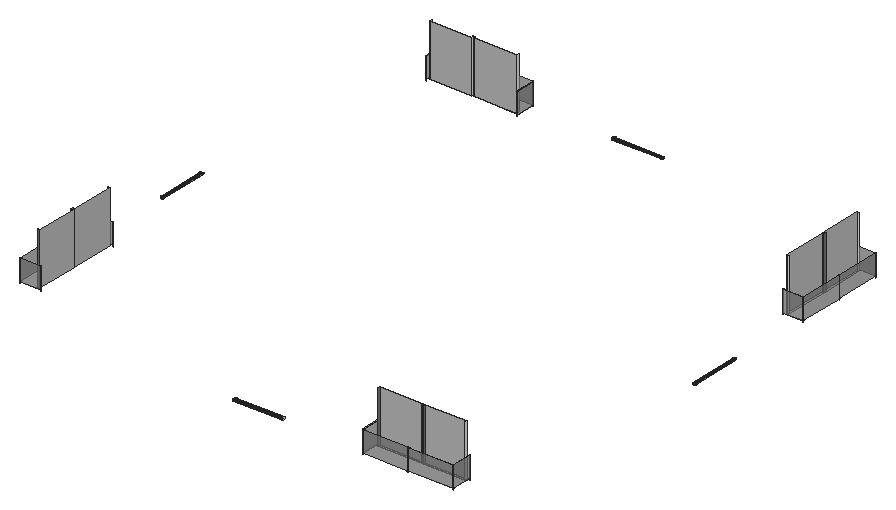
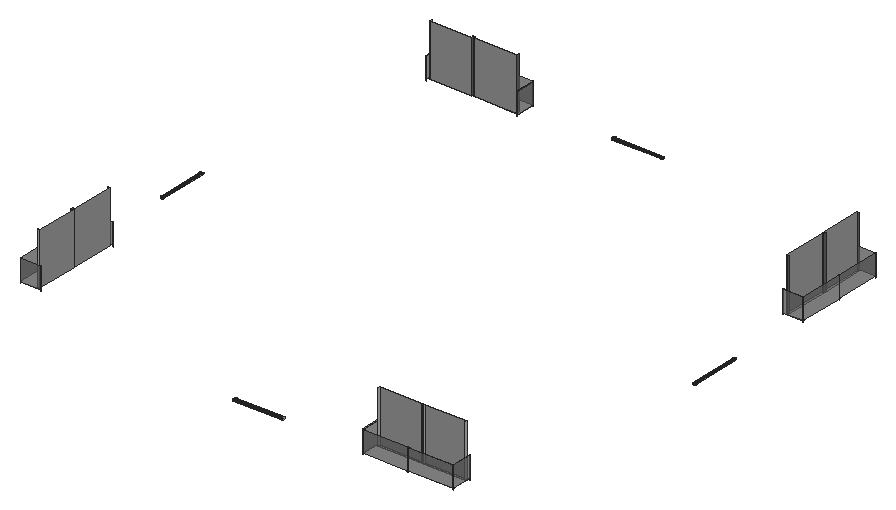
# SketchUp Ruby script. Lengths in inches.
U = 1.inch
M = Sketchup.active_model
def pt(a) = Geom::Point3d.new(a.map { |v| v * U })
def face(e, loops, mat)
  f = e.add_face(loops[0].map { |a| pt(a) })
  loops[1..].each { |l| e.add_face(l.map { |a| pt(a) }).erase! }
  f.material = f.back_material = mat if mat
  f
end
# faces: each face lists its corners as indices into pts; further lists are holes
def faces(e, pts, list, mat = nil) = list.each { |f| face(e, (f[0].is_a?(Array) ? f : [f]).map { |l| l.map { |i| pts[i] } }, mat) }
# xy, xz, yz: faces in a plane at the given z, y or x. An outline is a flat list of corners, or four numbers for a rectangle; further outlines are holes
def ring(l) = l.size == 4 ? [[l[0], l[1]], [l[2], l[1]], [l[2], l[3]], [l[0], l[3]]] : l.each_slice(2).to_a
def flat(e, list, mat, &to3) = list.each { |f| face(e, (f[0].is_a?(Array) ? f : [f]).map { |l| ring(l).map { |u, v| to3.(u, v) } }, mat) }
def xy(e, z, list, mat = nil) = flat(e, list, mat) { |x, y| [x, y, z] }
def xz(e, y, list, mat = nil) = flat(e, list, mat) { |x, z| [x, y, z] }
def yz(e, x, list, mat = nil) = flat(e, list, mat) { |y, z| [x, y, z] }
def lines(e, pts, list) = list.each { |a, b| e.add_line(pt(pts[a]), pt(pts[b])) }
# prism: a flat outline (further loops are holes) pulled along v
def prism(e, loops, v, mat = nil)
  f = face(e, loops, mat); d = Geom::Vector3d.new(v.map { |x| x * U })
  f.pushpull(f.normal.samedirection?(d) ? d.length : -d.length)
end
def box(e, o, s, mat = nil) = prism(e, [[o, [o[0] + s[0], o[1], o[2]], [o[0] + s[0], o[1] + s[1], o[2]], [o[0], o[1] + s[1], o[2]]]], [0, 0, s[2]], mat)
def at(x, y, z, deg = 0) = Geom::Transformation.translation(pt([x, y, z])) * Geom::Transformation.rotation(ORIGIN, Z_AXIS, deg.degrees)
def axes(o, x, y, z) = Geom::Transformation.new([*x, 0, *y, 0, *z, 0, *pt(o).to_a, 1])
def part(name) = M.definitions.add(name)
# library, detail: a bought-in or finely detailed component or shape, given as its bounding box
def library(name, o, s) = part(name).tap { |d| box(d.entities, o, s) }
def detail(e, o, s) = box(e.add_group.entities, o, s)
def put(e, d, t, mat = nil) = e.add_instance(d, t).tap { |i| i.material = mat if mat }
def group(e, t, mat = nil) = e.add_group.tap { |g| g.transformation = t; g.material = mat if mat }.entities
root = M.entities
M.materials.add("[Metal Seamed]").color = [118, 119, 115]
M.materials.add("[Mirror 01]").color = [185, 185, 185]
M.materials.add("[Translucent Glass Tinted]").color = [8, 201, 241]
M.materials["[Translucent Glass Tinted]"].alpha = 0.48
M.materials.add("[Translucent_Glass_Gray]").color = [128, 128, 128]
M.materials["[Translucent_Glass_Gray]"].alpha = 0.5
c1 = part("Staal sojle alta")
box(c1.entities,[0,0,0],[0.87,0.87,43.31])
c2 = part("gler")
box(c2.entities,[0,-0.71,0],[0.37,57.8,41.34],"[Translucent_Glass_Gray]")
xy(root,859.11,[[1161.2,84.8125,1285.04,90.8125],[1291.04,84.8125,1408.89,90.8125],[120,175.92,126,293.77],[120,299.77,126,423.61],[1494,1126.01,1500,1249.86],
  [1494,1255.86,1500,1373.7],[211.11,1458.8125,328.96,1464.8125],[334.96,1458.8125,458.8,1464.8125]])
xz(root,84.8125,[[1285.04,859.11,1291.04,1007.61]],"[Metal Seamed]")
xz(root,90.8125,[[1161.2,859.11,1285.04,1007.61],[1291.04,859.11,1408.89,1007.61]],"[Mirror 01]")
xz(root,175.92,[[120,859.11,126,1007.61]],"[Metal Seamed]")
xz(root,293.77,[[120,859.11,126,1007.61]],"[Metal Seamed]")
xz(root,299.77,[[120,859.11,126,1007.61]],"[Metal Seamed]")
xz(root,423.61,[[120,859.11,126,1007.61]],"[Metal Seamed]")
xz(root,662.8,[[83.53,858.02,84.48,858.14,85.37,858.51,86.13,859.1,86.72,859.86,87.09,860.75,87.21,861.7,87.09,862.66,86.72,863.55,86.13,864.3125,85.37,864.9,84.48,865.27,83.53,865.39,82.57,865.27,81.68,864.9,80.92,864.3125,80.33,863.55,79.97,862.66,79.84,861.7,79.97,860.75,80.33,859.86,80.92,859.1,81.68,858.51,82.57,858.14]])
xz(root,886.83,[[1536.47,858.02,1535.52,858.14,1534.63,858.51,1533.87,859.1,1533.28,859.86,1532.91,860.75,1532.79,861.7,1532.91,862.66,1533.28,863.55,1533.87,864.3125,1534.63,864.9,1535.52,865.27,1536.47,865.39,1537.43,865.27,1538.32,864.9,1539.08,864.3125,1539.67,863.55,1540.03,862.66,1540.16,861.7,1540.03,860.75,1539.67,859.86,1539.08,859.1,1538.32,858.51,1537.43,858.14]])
xz(root,1126.01,[[1494,859.11,1500,1007.61]])
xz(root,1249.86,[[1494,859.11,1500,1007.61]])
xz(root,1255.86,[[1494,859.11,1500,1007.61]])
xz(root,1373.7,[[1494,859.11,1500,1007.61]])
xz(root,1458.8125,[[211.11,859.11,328.96,1007.61],[334.96,859.11,458.8,1007.61]],"[Mirror 01]")
xz(root,1464.8125,[[328.96,859.11,334.96,1007.61]],"[Metal Seamed]")
yz(root,120,[[293.77,859.11,299.77,1007.61]],"[Metal Seamed]")
yz(root,126,[[175.92,859.11,293.77,1007.61],[299.77,859.11,423.61,1007.61]],"[Mirror 01]")
yz(root,211.11,[[1458.8125,859.11,1464.8125,1007.61]])
yz(root,328.96,[[1458.8125,859.11,1464.8125,1007.61]])
yz(root,334.96,[[1458.8125,859.11,1464.8125,1007.61]])
yz(root,458.8,[[1458.8125,859.11,1464.8125,1007.61]])
yz(root,697.99,[[1501.28,858.02,1500.33,858.14,1499.44,858.51,1498.68,859.1,1498.09,859.86,1497.72,860.75,1497.6,861.7,1497.72,862.66,1498.09,863.55,1498.68,864.3125,1499.44,864.9,1500.33,865.27,1501.28,865.39,1502.24,865.27,1503.13,864.9,1503.89,864.3125,1504.48,863.55,1504.85,862.66,1504.97,861.7,1504.85,860.75,1504.48,859.86,1503.89,859.1,1503.13,858.51,1502.24,858.14]])
yz(root,922.01,[[48.34,858.02,49.29,858.14,50.18,858.51,50.95,859.1,51.53,859.86,51.9,860.75,52.03,861.7,51.9,862.66,51.53,863.55,50.95,864.3125,50.18,864.9,49.29,865.27,48.34,865.39,47.38,865.27,46.5,864.9,45.73,864.3125,45.15,863.55,44.78,862.66,44.65,861.7,44.78,860.75,45.15,859.86,45.73,859.1,46.5,858.51,47.38,858.14]])
yz(root,1161.2,[[84.8125,859.11,90.8125,1007.61]],"[Metal Seamed]")
yz(root,1285.04,[[84.8125,859.11,90.8125,1007.61]])
yz(root,1291.04,[[84.8125,859.11,90.8125,1007.61]],"[Metal Seamed]")
yz(root,1408.89,[[84.8125,859.11,90.8125,1007.61]])
yz(root,1494,[[1126.01,859.11,1249.86,1007.61],[1255.86,859.11,1373.7,1007.61]],"[Mirror 01]")
yz(root,1500,[[1249.86,859.11,1255.86,1007.61]],"[Metal Seamed]")
p = [[922.01,48.34,858.02],[922.01,47.38,858.14],[778.64,47.38,858.14],[778.64,48.34,858.02],[922.01,49.29,858.14],[778.64,49.29,858.14],
  [83.53,662.8,858.02],[82.57,662.8,858.14],[82.57,806.17,858.14],[83.53,806.17,858.02],[84.48,662.8,858.14],[84.48,806.17,858.14],
  [1535.52,886.83,858.14],[1536.47,886.83,858.02],[1536.47,743.45,858.02],[1535.52,743.45,858.14],[1537.43,886.83,858.14],[1537.43,743.45,858.14],
  [697.99,1500.33,858.14],[697.99,1501.28,858.02],[841.36,1501.28,858.02],[841.36,1500.33,858.14],[697.99,1502.24,858.14],[841.36,1502.24,858.14],
  [922.01,46.5,858.51],[778.64,46.5,858.51],[922.01,50.18,858.51],[778.64,50.18,858.51],[81.68,662.8,858.51],[81.68,806.17,858.51],
  [85.37,662.8,858.51],[85.37,806.17,858.51],[1534.63,886.83,858.51],[1534.63,743.45,858.51],[1538.32,886.83,858.51],[1538.32,743.45,858.51],
  [697.99,1499.44,858.51],[841.36,1499.44,858.51],[697.99,1503.13,858.51],[841.36,1503.13,858.51],[922.01,45.73,859.1],[778.64,45.73,859.1],
  [922.01,50.95,859.1],[778.64,50.95,859.1],[80.92,662.8,859.1],[80.92,806.17,859.1],[86.13,662.8,859.1],[86.13,806.17,859.1],
  [1533.87,886.83,859.1],[1533.87,743.45,859.1],[1539.08,886.83,859.1],[1539.08,743.45,859.1],[697.99,1498.68,859.1],[841.36,1498.68,859.1],
  [697.99,1503.89,859.1],[841.36,1503.89,859.1],[922.01,45.15,859.86],[778.64,45.15,859.86],[922.01,51.53,859.86],[778.64,51.53,859.86],
  [80.33,662.8,859.86],[80.33,806.17,859.86],[86.72,662.8,859.86],[86.72,806.17,859.86],[1533.28,886.83,859.86],[1533.28,743.45,859.86],
  [1539.67,886.83,859.86],[1539.67,743.45,859.86],[697.99,1498.09,859.86],[841.36,1498.09,859.86],[697.99,1504.48,859.86],[841.36,1504.48,859.86],
  [922.01,44.78,860.75],[778.64,44.78,860.75],[922.01,51.9,860.75],[778.64,51.9,860.75],[79.97,662.8,860.75],[79.97,806.17,860.75],
  [87.09,662.8,860.75],[87.09,806.17,860.75],[1532.91,886.83,860.75],[1532.91,743.45,860.75],[1540.03,886.83,860.75],[1540.03,743.45,860.75],
  [697.99,1497.72,860.75],[841.36,1497.72,860.75],[697.99,1504.85,860.75],[841.36,1504.85,860.75],[922.01,44.65,861.7],[778.64,44.65,861.7],
  [922.01,52.03,861.7],[778.64,52.03,861.7],[79.84,662.8,861.7],[79.84,806.17,861.7],[87.21,662.8,861.7],[87.21,806.17,861.7],
  [1532.79,886.83,861.7],[1532.79,743.45,861.7],[1540.16,886.83,861.7],[1540.16,743.45,861.7],[697.99,1497.6,861.7],[841.36,1497.6,861.7],
  [697.99,1504.97,861.7],[841.36,1504.97,861.7],[922.01,44.78,862.66],[778.64,44.78,862.66],[922.01,51.9,862.66],[778.64,51.9,862.66],
  [79.97,662.8,862.66],[79.97,806.17,862.66],[87.09,662.8,862.66],[87.09,806.17,862.66],[1532.91,886.83,862.66],[1532.91,743.45,862.66],
  [1540.03,886.83,862.66],[1540.03,743.45,862.66],[697.99,1497.72,862.66],[841.36,1497.72,862.66],[697.99,1504.85,862.66],[841.36,1504.85,862.66],
  [922.01,45.15,863.55],[778.64,45.15,863.55],[922.01,51.53,863.55],[778.64,51.53,863.55],[80.33,662.8,863.55],[80.33,806.17,863.55],
  [86.72,662.8,863.55],[86.72,806.17,863.55],[1533.28,886.83,863.55],[1533.28,743.45,863.55],[1539.67,886.83,863.55],[1539.67,743.45,863.55],
  [697.99,1498.09,863.55],[841.36,1498.09,863.55],[697.99,1504.48,863.55],[841.36,1504.48,863.55],[697.99,1501.28,861.7],[841.36,1501.28,861.7],
  [1536.47,886.83,861.7],[1536.47,743.45,861.7],[922.01,48.34,861.7],[778.64,48.34,861.7],[83.53,662.8,861.7],[83.53,806.17,861.7]]
faces(root,p,[[0,1,2,3],[4,0,3,5],[6,7,8,9],[10,6,9,11],[12,13,14,15],[13,16,17,14],[18,19,20,21],[19,22,23,20],
  [1,24,25,2],[26,4,5,27],[7,28,29,8],[30,10,11,31],[32,12,15,33],[16,34,35,17],[36,18,21,37],[22,38,39,23],
  [24,40,41,25],[42,26,27,43],[28,44,45,29],[46,30,31,47],[48,32,33,49],[34,50,51,35],[52,36,37,53],[38,54,55,39],
  [40,56,57,41],[58,42,43,59],[44,60,61,45],[62,46,47,63],[64,48,49,65],[50,66,67,51],[68,52,53,69],[54,70,71,55],
  [56,72,73,57],[74,58,59,75],[60,76,77,61],[78,62,63,79],[80,64,65,81],[66,82,83,67],[84,68,69,85],[70,86,87,71],
  [72,88,89,73],[90,74,75,91],[76,92,93,77],[94,78,79,95],[96,80,81,97],[82,98,99,83],[100,84,85,101],[86,102,103,87],
  [88,104,105,89],[106,90,91,107],[92,108,109,93],[110,94,95,111],[112,96,97,113],[98,114,115,99],[116,100,101,117],[102,118,119,103],
  [104,120,121,105],[122,106,107,123],[108,124,125,109],[126,110,111,127],[128,112,113,129],[114,130,131,115],[132,116,117,133],[118,134,135,119]])
lines(root,p,[[136,137],[138,139],[140,141],[142,143]])
put(root,c1,axes([1487.13,1121.96,855.08],[0,-2.19843,0],[1,0,0],[0,0,1.5]),"[Translucent Glass Tinted]")
put(root,c1,axes([1545.31,1250.93,855.08],[0,-2.19843,0],[1,0,0],[0,0,1.5]),"[Translucent Glass Tinted]")
put(root,c1,axes([74.69,298.69,855.08],[0,2.19843,0],[-1,0,0],[0,0,1.5]),"[Translucent Glass Tinted]")
put(root,c1,axes([462.85,1510.125,855.08],[2.19843,0,0],[0,1,0],[0,0,1.5]),"[Translucent Glass Tinted]")
put(root,c1,axes([205.11,1451.94,855.08],[2.19843,0,0],[0,1,0],[0,0,1.5]),"[Translucent Glass Tinted]")
put(root,c1,axes([1414.89,39.5,855.08],[-2.19843,0,0],[0,-1,0],[0,0,1.5]),"[Translucent Glass Tinted]")
put(root,c1,axes([1286.12,39.5,855.08],[-2.19843,0,0],[0,-1,0],[0,0,1.5]),"[Translucent Glass Tinted]")
put(root,c1,axes([205.11,1510.125,855.08],[2.19843,0,0],[0,1,0],[0,0,1.5]),"[Translucent Glass Tinted]")
put(root,c1,axes([74.69,427.66,855.08],[0,2.19843,0],[-1,0,0],[0,0,1.5]),"[Translucent Glass Tinted]")
put(root,c1,axes([74.69,169.92,855.08],[0,2.19843,0],[-1,0,0],[0,0,1.5]),"[Translucent Glass Tinted]")
put(root,c1,axes([132.87,169.92,855.08],[0,2.19843,0],[-1,0,0],[0,0,1.5]),"[Translucent Glass Tinted]")
put(root,c1,axes([1157.15,97.68,855.08],[-2.19843,0,0],[0,-1,0],[0,0,1.5]),"[Translucent Glass Tinted]")
put(root,c1,axes([132.87,427.66,855.08],[0,2.19843,0],[-1,0,0],[0,0,1.5]),"[Translucent Glass Tinted]")
put(root,c1,axes([462.85,1451.94,855.08],[2.19843,0,0],[0,1,0],[0,0,1.5]),"[Translucent Glass Tinted]")
put(root,c1,axes([1414.89,97.68,855.08],[-2.19843,0,0],[0,-1,0],[0,0,1.5]),"[Translucent Glass Tinted]")
put(root,c1,axes([333.88,1510.125,855.08],[2.19843,0,0],[0,1,0],[0,0,1.5]),"[Translucent Glass Tinted]")
put(root,c1,axes([1545.31,1379.7,855.08],[0,-2.19843,0],[1,0,0],[0,0,1.5]),"[Translucent Glass Tinted]")
put(root,c1,axes([1545.31,1121.96,855.08],[0,-2.19843,0],[1,0,0],[0,0,1.5]),"[Translucent Glass Tinted]")
put(root,c1,axes([1157.15,39.5,855.08],[-2.19843,0,0],[0,-1,0],[0,0,1.5]),"[Translucent Glass Tinted]")
put(root,c1,axes([1487.13,1379.7,855.08],[0,-2.19843,0],[1,0,0],[0,0,1.5]),"[Translucent Glass Tinted]")
put(root,c2,axes([1488.23,1379.7,858.03],[0,-2.19843,0],[1,0,0],[0,0,1.5]),"[Translucent Glass Tinted]")
put(root,c2,axes([464.03,1453.04,858.03],[2.19843,0,0],[0,1,0],[0,0,1.5]),"[Translucent Glass Tinted]")
put(root,c2,axes([337.35,1511,858.03],[0,-1,0],[2.19843,0,0],[0,0,1.5]),"[Translucent Glass Tinted]")
put(root,c2,axes([1411.62,38.625,858.03],[0,1,0],[-2.19843,0,0],[0,0,1.5]),"[Translucent Glass Tinted]")
put(root,c2,axes([131.77,428.84,858.03],[0,2.19843,0],[-1,0,0],[0,0,1.5]),"[Translucent Glass Tinted]")
put(root,c2,axes([1155.97,96.58,858.03],[-2.19843,0,0],[0,-1,0],[0,0,1.5]),"[Translucent Glass Tinted]")
put(root,c2,axes([205.11,1453.04,858.03],[2.19843,0,0],[0,1,0],[0,0,1.5]),"[Translucent Glass Tinted]")
put(root,c2,axes([73.81,173.19,858.03],[1,0,0],[0,2.19843,0],[0,0,1.5]),"[Translucent Glass Tinted]")
put(root,c2,axes([1282.65,38.625,858.03],[0,1,0],[-2.19843,0,0],[0,0,1.5]),"[Translucent Glass Tinted]")
put(root,c2,axes([131.77,169.92,858.03],[0,2.19843,0],[-1,0,0],[0,0,1.5]),"[Translucent Glass Tinted]")
put(root,c2,axes([73.81,302.16,858.03],[1,0,0],[0,2.19843,0],[0,0,1.5]),"[Translucent Glass Tinted]")
put(root,c2,axes([208.38,1511,858.03],[0,-1,0],[2.19843,0,0],[0,0,1.5]),"[Translucent Glass Tinted]")
put(root,c2,axes([1414.89,96.58,858.03],[-2.19843,0,0],[0,-1,0],[0,0,1.5]),"[Translucent Glass Tinted]")
put(root,c2,axes([1488.23,1120.78,858.03],[0,-2.19843,0],[1,0,0],[0,0,1.5]),"[Translucent Glass Tinted]")
put(root,c2,axes([1546.19,1376.43,858.03],[-1,0,0],[0,-2.19843,0],[0,0,1.5]),"[Translucent Glass Tinted]")
put(root,c2,axes([1546.19,1247.46,858.03],[-1,0,0],[0,-2.19843,0],[0,0,1.5]),"[Translucent Glass Tinted]")
